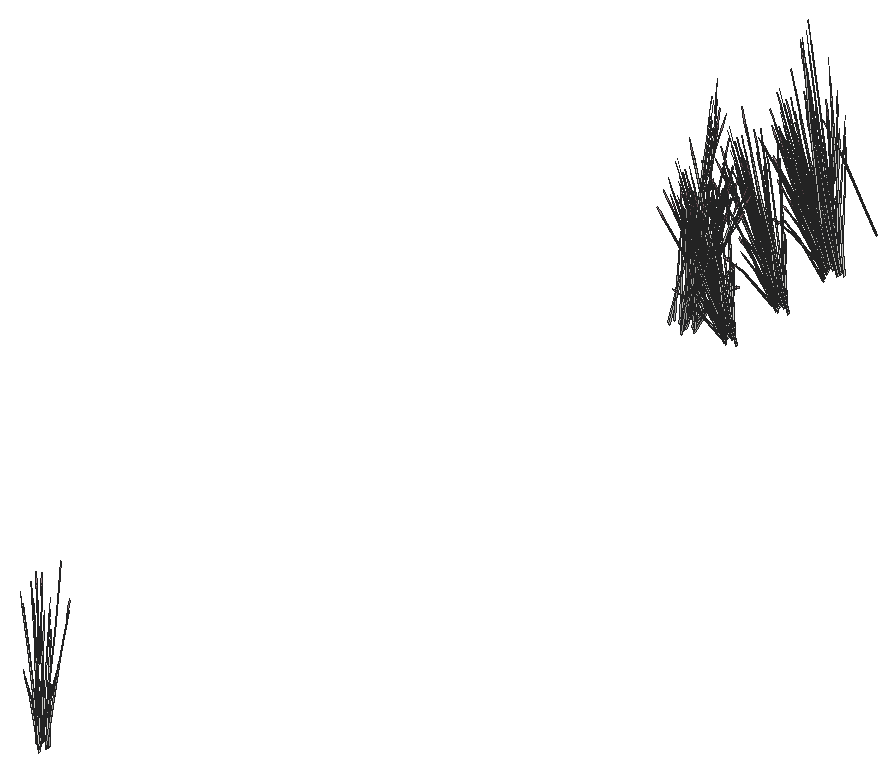
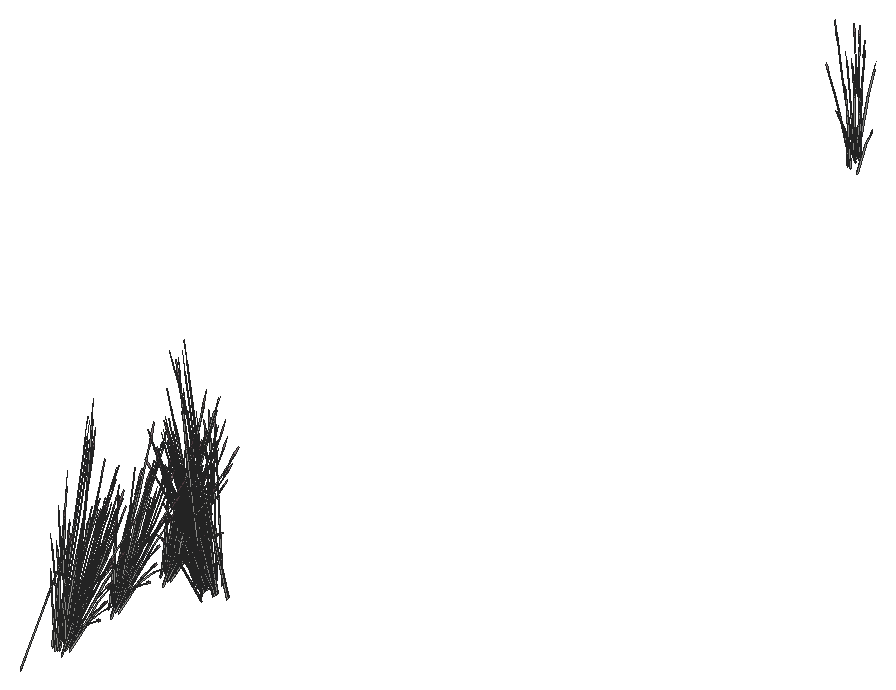
# SketchUp Ruby script. Lengths in inches.
U = 1.inch
M = Sketchup.active_model
def pt(a) = Geom::Point3d.new(a.map { |v| v * U })
def face(e, loops, mat)
  f = e.add_face(loops[0].map { |a| pt(a) })
  loops[1..].each { |l| e.add_face(l.map { |a| pt(a) }).erase! }
  f.material = f.back_material = mat if mat
  f
end
# faces: each face lists its corners as indices into pts; further lists are holes
def faces(e, pts, list, mat = nil) = list.each { |f| face(e, (f[0].is_a?(Array) ? f : [f]).map { |l| l.map { |i| pts[i] } }, mat) }
# xy, xz, yz: faces in a plane at the given z, y or x. An outline is a flat list of corners, or four numbers for a rectangle; further outlines are holes
def ring(l) = l.size == 4 ? [[l[0], l[1]], [l[2], l[1]], [l[2], l[3]], [l[0], l[3]]] : l.each_slice(2).to_a
def flat(e, list, mat, &to3) = list.each { |f| face(e, (f[0].is_a?(Array) ? f : [f]).map { |l| ring(l).map { |u, v| to3.(u, v) } }, mat) }
def xy(e, z, list, mat = nil) = flat(e, list, mat) { |x, y| [x, y, z] }
def xz(e, y, list, mat = nil) = flat(e, list, mat) { |x, z| [x, y, z] }
def yz(e, x, list, mat = nil) = flat(e, list, mat) { |y, z| [x, y, z] }
def lines(e, pts, list) = list.each { |a, b| e.add_line(pt(pts[a]), pt(pts[b])) }
# prism: a flat outline (further loops are holes) pulled along v
def prism(e, loops, v, mat = nil)
  f = face(e, loops, mat); d = Geom::Vector3d.new(v.map { |x| x * U })
  f.pushpull(f.normal.samedirection?(d) ? d.length : -d.length)
end
def box(e, o, s, mat = nil) = prism(e, [[o, [o[0] + s[0], o[1], o[2]], [o[0] + s[0], o[1] + s[1], o[2]], [o[0], o[1] + s[1], o[2]]]], [0, 0, s[2]], mat)
def at(x, y, z, deg = 0) = Geom::Transformation.translation(pt([x, y, z])) * Geom::Transformation.rotation(ORIGIN, Z_AXIS, deg.degrees)
def axes(o, x, y, z) = Geom::Transformation.new([*x, 0, *y, 0, *z, 0, *pt(o).to_a, 1])
def part(name) = M.definitions.add(name)
# library, detail: a bought-in or finely detailed component or shape, given as its bounding box
def library(name, o, s) = part(name).tap { |d| box(d.entities, o, s) }
def detail(e, o, s) = box(e.add_group.entities, o, s)
def put(e, d, t, mat = nil) = e.add_instance(d, t).tap { |i| i.material = mat if mat }
def group(e, t, mat = nil) = e.add_group.tap { |g| g.transformation = t; g.material = mat if mat }.entities
root = M.entities
M.materials.add("LightPink_Translucent").color = [144, 107, 117]
M.materials["LightPink_Translucent"].alpha = 0.75
c1 = part("blade")
p = [[2.15,0.21,22],[0,0.17,0],[0.09,0.45,0],[2.18,0.31,22],[2.29,0.31,22],[0.38,0.45,0],
  [2.48,0.24,33],[2.49,0.24,33],[2.48,0.22,33]]
faces(c1.entities,p,[[0,1,2,3],[4,5,2,3],[6,3,4,7],[8,0,3,6]])
c2 = part("seeds")
p = [[0.3,-0.1,1.38],[-0.01,-0.03,1.59],[-0.01,-0.03,0.03],[0.14,-0.07,-0.07],[0.29,-0.03,3],[0.15,0.01,3.11]]
faces(c2.entities,p,[[0,1,2,3],[1,0,4,5]],"LightPink_Translucent")
c3 = part("blade with seeds")
put(c3.entities,c1,at(0,0,0))
put(c3.entities,c2,axes([2.4,0.25,30.99],[1.5799,-0.05474,1.17369],[-0.12525,1.92788,0.29478],[-0.07173,-0.02425,1.56792]))
put(root,c3,axes([503.15,211.2,4.23],[0.70283,0.33692,-0.1216],[-0.40491,0.48793,-0.67495],[-0.19857,0.16961,1.02557]))
put(root,c3,axes([504.1,211.05,3.07],[0.18977,-0.18775,1.71376],[0.47917,0.50677,0.13857],[-0.32866,0.23079,0.73262]))
put(root,c3,axes([503.5,211.6,3.875],[0.19519,0.55794,-0.51099],[-0.73919,0.0976,-0.3958],[-0.21183,0.14986,0.97773]))
put(root,c3,axes([503.92,212.54,3.92],[-0.62439,-0.02847,0.0643],[0.01712,-0.42991,0.50621],[-0.06534,0.16468,0.77189]))
put(root,c3,axes([502.6,213.03,0.6875],[0.10192,0.06105,1.76342],[0.17281,0.56562,-0.26939],[-0.22588,0.12062,0.30037]))
put(root,c3,axes([504.12,212.57,3.93],[-0.54105,-0.41691,0.48003],[0.57458,-0.35956,0.3958],[-0.0998,0.1956,0.9933]))
put(root,c3,axes([503.96,211.52,3.07],[0.14147,-0.21002,1.71376],[0.59349,0.43464,0.13857],[-0.26773,0.27089,0.73262]))
put(root,c3,axes([504.12,212.7,3.72],[-0.5141,0.32171,-0.35414],[-0.48666,-0.36734,0.4572],[-0.07405,0.18664,0.87481]))
put(root,c3,axes([502.35,212.6,3.91],[-0.01889,0.12092,1.74944],[0.53598,0.42065,-0.27667],[-0.14032,0.19892,0.14031]))
put(root,c3,axes([504.45,213.95,1.96],[-0.01966,-0.36332,1.1486],[0.49135,0.25914,0.84392],[-0.09663,0.17317,0.25299]))
put(root,c3,axes([504.46,212.36,4.53],[-0.01977,0.56521,-0.7886],[-0.83252,-0.03796,0.09517],[-0.08786,0.23945,1.11556]))
put(root,c3,axes([502.29,213.84,3.9],[0.0862,-0.03689,1.77383],[0.71245,0.24539,-0.16761],[-0.01674,0.20431,0.31391]))
put(root,c3,axes([503.875,213.63,1.78],[0.23977,-0.09639,1.43002],[0.59198,0.29065,-0.30754],[-0.1762,0.25149,0.61141]))
put(root,c3,axes([504.19,213.16,2.56],[0.01669,-0.31544,1.54345],[0.75083,0.16661,0.21329],[-0.06506,0.33618,0.72882]))
put(root,c3,axes([493.98,440.93,3.07],[-0.14147,0.21002,1.71376],[-0.59349,-0.43464,0.13857],[0.26773,-0.27089,0.73262]))
put(root,c3,axes([508.48,440.87,4.17],[-0.64788,-0.29534,-0.71045],[0.46044,-0.51755,0.08574],[-0.23473,-0.17635,1.00501]))
put(root,c3,axes([506.8125,441.19,3.07],[0.28223,0.10528,1.71376],[-0.58406,0.44165,0.13857],[-0.36402,-0.19924,0.73262]))
put(root,c3,axes([495.9,440.68,0.6875],[-0.11372,-0.04814,1.76342],[-0.29211,-0.53779,-0.26939],[0.19706,-0.14594,0.30037]))
put(root,c3,axes([508.18,440.88,3.875],[-0.74975,0.14525,-0.51099],[-0.13115,-0.55007,-0.3958],[-0.20138,-0.15763,0.97773]))
put(root,c3,axes([495.25,441,3.93],[0.54105,0.41691,0.48003],[-0.57458,0.35956,0.3958],[0.0998,-0.1956,0.9933]))
put(root,c3,axes([508.7,440.39,4.62],[-0.50709,0.58578,-0.13619],[-0.73436,-0.33748,-0.75594],[-0.25527,-0.1655,1.14864]))
put(root,c3,axes([495.89,442.2,4.17],[0.39688,-0.48213,-0.71045],[0.69548,0.34264,0.08574],[0.23697,-0.17468,1.00501]))
put(root,c3,axes([495.875,441.97,3.875],[-0.19519,-0.55794,-0.51099],[0.73919,-0.0976,-0.3958],[0.21183,-0.14986,0.97773]))
put(root,c3,axes([506.76,440.22,3.91],[-0.16348,-0.00431,1.74944],[-0.52047,0.43131,-0.27667],[-0.2777,-0.08813,0.14031]))
put(root,c3,axes([496.22,442.37,4.23],[-0.70283,-0.33692,-0.1216],[0.40491,-0.48793,-0.67495],[0.19857,-0.16961,1.02557]))
put(root,c3,axes([496.47,441.75,1.78],[-0.27143,-0.0181,1.43002],[-0.27808,-0.48551,-0.30754],[0.33346,-0.13735,0.61141]))
put(root,c3,axes([506.64,441.2,4.29],[0.62747,-0.45094,0.53763],[0.54116,0.47889,0.4433],[-0.29439,-0.08318,1.11249]))
put(root,c3,axes([497.95,442.22,3.9],[-0.09924,-0.00464,1.77383],[-0.4121,-0.49725,-0.16761],[0.1655,-0.1635,0.31391]))
put(root,c3,axes([496.78,440.86,1.96],[-0.25308,0.31105,1.1486],[-0.21753,-0.4179,0.84392],[0.20902,-0.10472,0.25299]))
put(root,c3,axes([496.42,442.03,3.72],[0.66138,-0.08733,-0.35414],[0.17464,0.49921,0.4572],[0.18953,-0.13408,0.87481]))
put(root,c3,axes([506.92,441.2,3.92],[0.03826,-0.46465,0.0643],[0.57772,0.01274,0.50621],[-0.2213,-0.04862,0.77189]))
put(root,c3,axes([506.7,441.34,3.72],[-0.43232,-0.38257,-0.35414],[0.49364,-0.36215,0.4572],[-0.25081,-0.0551,0.87481]))
put(root,c3,axes([495.88,442.32,4.24],[-0.66138,0.08733,0.35414],[-0.17464,-0.49921,-0.4572],[0.18953,-0.13408,0.87481]))
put(root,c3,axes([506.55,441.75,1.78],[0.14835,0.17012,1.43002],[-0.34183,0.46242,-0.30754],[-0.351,-0.11053,0.61141]))
put(root,c3,axes([507.16,441.6,4.17],[-0.75952,-0.01471,-0.71045],[0.05101,-0.61953,0.08574],[-0.32177,-0.06538,1.00501]))
put(root,c3,axes([496.48,442.25,3.92],[0.52161,0.25698,0.0643],[-0.30368,0.36595,0.50621],[0.16723,-0.11831,0.77189]))
put(root,c3,axes([496.33,442.14,3.93],[0.18844,0.56237,0.48003],[-0.73919,0.0976,0.3958],[0.21785,-0.13226,0.9933]))
put(root,c3,axes([498.33,442.82,3.91],[0.10543,-0.09307,1.74944],[-0.13495,-0.57092,-0.27667],[0.26455,-0.10825,0.14031]))
put(root,c3,axes([506.13,440.59,3.9],[0.05633,0.06098,1.77383],[-0.27155,0.54815,-0.16761],[-0.27501,0.00397,0.31391]))
put(root,c3,axes([506.91,441.72,3.875],[-0.55171,0.40476,-0.51099],[-0.48318,-0.42758,-0.3958],[-0.28031,-0.06159,0.97773]))
put(root,c3,axes([507.31,441.54,4.24],[0.43232,0.38257,0.35414],[-0.49364,0.36215,-0.4572],[-0.25081,-0.0551,0.87481]))
put(root,c3,axes([505.66,442.26,1.96],[0.48508,-0.04372,1.1486],[-0.3077,0.38525,0.84392],[-0.23971,-0.05779,0.25299]))
put(root,c3,axes([507.2,441.3,4.23],[-0.04068,0.62141,-0.1216],[-0.77029,-0.01698,-0.67495],[-0.29667,-0.04317,1.02557]))
put(root,c3,axes([496.25,443.69,4.23],[-0.38229,-0.5533,-0.1216],[0.6785,-0.2719,-0.67495],[0.28593,-0.073,1.02557]))
put(root,c3,axes([496.22,443.21,3.875],[0.20584,-0.55581,-0.51099],[0.70573,0.19051,-0.3958],[0.28414,-0.05097,0.97773]))
put(root,c3,axes([495.1,440.95,1.57],[0.47504,-0.61229,0],[0.79476,0.34146,-0.51607],[0.18101,0.07777,1.63711]))
put(root,c3,axes([506.22,442.16,3.07],[0.31515,-0.01384,1.71376],[-0.20907,0.5998,0.13857],[-0.44912,-0.0371,0.73262]))
put(root,c3,axes([496.97,443.37,1.17],[-0.48937,0.07333,1.41583],[-0.07789,-0.58369,0.08104],[0.34275,-0.08835,0.80566]))
put(root,c3,axes([497.86,442.85,1.45],[-0.47106,-0.39072,-0.06488],[0.51591,-0.35801,-0.29416],[0.14618,-0.02521,0.97024]))
put(root,c3,axes([496.08,443.41,4.17],[0.66765,-0.26986,-0.71045],[0.37208,0.55551,0.08574],[0.32259,-0.0631,1.00501]))
put(root,c3,axes([508.56,443.76,1.25],[-0.79037,-0.10018,-0.62353],[0.16679,-0.61794,-0.16365],[-0.23587,-0.07488,1.37633]))
put(root,c3,axes([495.98,443.52,4.24],[-0.63144,-0.17046,0.35414],[0.18417,-0.49731,-0.4572],[0.25423,-0.0456,0.87481]))
put(root,c3,axes([506.09,442.61,3.93],[0.21466,-0.55714,0.48003],[0.70573,0.19051,0.3958],[-0.27753,0.03348,0.9933]))
put(root,c3,axes([491.66,442.03,0.79],[-0.74787,0.24464,1.28929],[-0.23804,-0.70192,0.50096],[0.45924,0.01168,1.46642]))
put(root,c3,axes([506.03,442.46,3.92],[-0.27906,-0.41663,0.0643],[0.50888,-0.20393,0.50621],[-0.22432,0.04024,0.77189]))
put(root,c3,axes([497.5,442.98,0.6875],[-0.03971,-0.09277,1.76342],[0.27541,-0.54264,-0.26939],[0.27782,-0.00781,0.30037]))
put(root,c3,axes([506.02,442.89,0.6875],[0.01927,0.0963,1.76342],[-0.38846,0.5029,-0.26939],[-0.27592,-0.02535,0.30037]))
put(root,c3,axes([493.6,442.39,1.86],[0.76714,-0.40567,-0.29095],[0.51013,0.57321,-0.50002],[0.18927,0.05821,1.59708]))
put(root,c3,axes([496.65,443.46,3.72],[0.63144,0.17046,-0.35414],[-0.18417,0.49731,0.4572],[0.25423,-0.0456,0.87481]))
put(root,c3,axes([495.53,441.32,1.21],[0.7111,0.30552,-0.49651],[-0.42504,0.54784,0],[0.16196,0.06958,1.57504]))
put(root,c3,axes([505.9375,442.67,3.72],[-0.63144,-0.17046,-0.35414],[0.18417,-0.49731,0.4572],[-0.25423,0.0456,0.87481]))
put(root,c3,axes([494.93,442.85,3.07],[-0.31515,0.01384,1.71376],[0.20907,-0.5998,0.13857],[0.44912,0.0371,0.73262]))
put(root,c3,axes([495.34,441.54,1.22],[0.17848,0.53243,-0.30978],[-0.70886,0.15119,0.30978],[0.1429,0.0614,1.38974]))
put(root,c3,axes([496.56,443.67,3.92],[0.27906,0.41663,0.0643],[-0.50888,0.20393,0.50621],[0.22432,-0.04024,0.77189]))
put(root,c3,axes([496.5,443.52,3.93],[-0.21466,0.55714,0.48003],[-0.70573,-0.19051,0.3958],[0.27753,-0.03348,0.9933]))
put(root,c3,axes([506.6,442.62,4.24],[0.63144,0.17046,0.35414],[-0.18417,0.49731,-0.4572],[-0.25423,0.0456,0.87481]))
put(root,c3,axes([507.86,442.59,2.53],[0.21597,-0.08839,1.77064],[0.07448,0.61717,0.13857],[-0.4678,0.08189,0.63284]))
put(root,c3,axes([494.5,442.49,1.25],[0.79037,0.10018,-0.62353],[-0.16679,0.61794,-0.16365],[0.23587,0.07488,1.37633]))
put(root,c3,axes([497.99,443.56,1.96],[-0.46945,0.10088,1.1486],[0.22097,-0.4169,0.84392],[0.24904,0.02853,0.25299]))
put(root,c3,axes([497.77,445.33,3.9],[-0.0687,-0.05349,1.77383],[0.15029,-0.57341,-0.16761],[0.27062,-0.03664,0.31391]))
put(root,c3,axes([505.54,443,3.91],[-0.12407,0.07933,1.74944],[0.01055,0.57963,-0.27667],[-0.2844,0.07538,0.14031]))
put(root,c3,axes([506.37,442.92,3.875],[-0.20584,0.55581,-0.51099],[-0.70573,-0.19051,-0.3958],[-0.28414,0.05097,0.97773]))
put(root,c3,axes([506.34,442.45,4.23],[0.38229,0.5533,-0.1216],[-0.6785,0.2719,-0.67495],[-0.28593,0.073,1.02557]))
put(root,c3,axes([497.17,444.85,3.12],[-0.14542,-0.51365,-0.03492],[0.68734,-0.11809,-0.15832],[0.14353,0.03256,0.52218]))
put(root,c3,axes([495.39,444.83,4.23],[0.04068,-0.62141,-0.1216],[0.77029,0.01698,-0.67495],[0.29667,0.04317,1.02557]))
put(root,c3,axes([495.27,444.59,4.24],[-0.43232,-0.38257,0.35414],[0.49364,-0.36215,-0.4572],[0.25081,0.0551,0.87481]))
put(root,c3,axes([496.0625,444.46,3.91],[0.16299,-0.01033,1.74944],[0.44707,-0.47471,-0.27667],[0.28992,0.06266,0.14031]))
put(root,c3,axes([506.26,444,3.93],[-0.18844,-0.56237,0.48003],[0.73919,-0.0976,0.3958],[-0.21785,0.13226,0.9933]))
put(root,c3,axes([506.11,443.89,3.92],[-0.52161,-0.25698,0.0643],[0.30368,-0.36595,0.50621],[-0.16723,0.11831,0.77189]))
put(root,c3,axes([506.35,443.21,3.07],[0.26363,-0.12925,1.71376],[0.22195,0.59723,0.13857],[-0.41388,0.13498,0.73262]))
put(root,c3,axes([495.43,444.54,4.17],[0.75952,0.01471,-0.71045],[-0.05101,0.61953,0.08574],[0.32177,0.06538,1.00501]))
put(root,c3,axes([505.53,444.23,1.78],[0.26405,0.05016,1.43002],[0.17019,0.51235,-0.30754],[-0.35868,0.0959,0.61141]))
put(root,c3,axes([496.67,443.28,1.57],[0.95008,0,0],[0,0.68292,-0.51607],[0,0.15554,1.63711]))
put(root,c3,axes([504.16,443.59,3.9],[0.09697,0.01639,1.77383],[0.29997,0.53988,-0.16761],[-0.1985,0.1417,0.31391]))
put(root,c3,axes([504.98,445.3,1.96],[0.31665,-0.27694,1.1486],[0.12495,0.43841,0.84392],[-0.22883,0.0785,0.25299]))
put(root,c3,axes([495.89,444.79,3.72],[0.43232,0.38257,-0.35414],[-0.49364,0.36215,0.4572],[0.25081,0.0551,0.87481]))
put(root,c3,axes([495.67,444.9375,3.92],[-0.03826,0.46465,0.0643],[-0.57772,-0.01274,0.50621],[0.2213,0.04862,0.77189]))
put(root,c3,axes([506.17,444.11,3.72],[-0.66138,0.08733,-0.35414],[-0.17464,-0.49921,0.4572],[-0.18953,0.13408,0.87481]))
put(root,c3,axes([495.72,444.79,3.93],[-0.56024,0.40262,0.48003],[-0.48318,-0.42758,0.3958],[0.26285,0.07427,0.9933]))
put(root,c3,axes([494.33,443.81,3.07],[-0.28223,-0.10528,1.71376],[0.58406,-0.44165,0.13857],[0.36402,0.19924,0.73262]))
put(root,c3,axes([493.875,445.51,4.23],[0.45276,-0.52302,-0.1216],[0.65568,0.30132,-0.67495],[0.22792,0.14777,1.02557]))
put(root,c3,axes([507.3125,443.61,3.07],[0.18977,-0.18775,1.71376],[0.47917,0.50677,0.13857],[-0.32866,0.23079,0.73262]))
put(root,c3,axes([506.71,444.16,3.875],[0.19519,0.55794,-0.51099],[-0.73919,0.0976,-0.3958],[-0.21183,0.14986,0.97773]))
put(root,c3,axes([495.5,445.66,0.6875],[0.05536,-0.08822,1.76342],[0.69692,-0.25981,-0.26939],[0.21129,0.13447,0.30037]))
put(root,c3,axes([505.81,445.59,0.6875],[0.10192,0.06105,1.76342],[0.17281,0.56562,-0.26939],[-0.22588,0.12062,0.30037]))
put(root,c3,axes([494.41,445.25,3.875],[0.74975,-0.14525,-0.51099],[0.13115,0.55007,-0.3958],[0.20138,0.15763,0.97773]))
put(root,c3,axes([495.45,445.81,1.86],[-0.48723,-0.01916,1.0506],[0.32177,-0.40701,0.58006],[0.19248,0.1446,0.8241]))
put(root,c3,axes([507.17,444.08,3.07],[0.14147,-0.21002,1.71376],[0.59349,0.43464,0.13857],[-0.26773,0.27089,0.73262]))
put(root,c3,axes([505.5625,445.17,3.91],[-0.01889,0.12092,1.74944],[0.53598,0.42065,-0.27667],[-0.14032,0.19892,0.14031]))
put(root,c3,axes([508.59,458.49,4.17],[-0.64788,-0.29534,-0.71045],[0.46044,-0.51755,0.08574],[-0.23473,-0.17635,1.00501]))
put(root,c3,axes([506.93,458.8125,3.07],[0.28223,0.10528,1.71376],[-0.58406,0.44165,0.13857],[-0.36402,-0.19924,0.73262]))
put(root,c3,axes([508.81,458.01,4.62],[-0.50709,0.58578,-0.13619],[-0.73436,-0.33748,-0.75594],[-0.25527,-0.1655,1.14864]))
put(root,c3,axes([506.87,457.84,3.91],[-0.16348,-0.00431,1.74944],[-0.52047,0.43131,-0.27667],[-0.2777,-0.08813,0.14031]))
put(root,c3,axes([506.75,458.82,4.29],[0.62747,-0.45094,0.53763],[0.54116,0.47889,0.4433],[-0.29439,-0.08318,1.11249]))
put(root,c3,axes([507.04,458.81,3.92],[0.03826,-0.46465,0.0643],[0.57772,0.01274,0.50621],[-0.2213,-0.04862,0.77189]))
put(root,c3,axes([506.82,458.96,3.72],[-0.43232,-0.38257,-0.35414],[0.49364,-0.36215,0.4572],[-0.25081,-0.0551,0.87481]))
put(root,c3,axes([506.66,459.37,1.78],[0.14835,0.17012,1.43002],[-0.34183,0.46242,-0.30754],[-0.351,-0.11053,0.61141]))
put(root,c3,axes([507.27,459.22,4.17],[-0.75952,-0.01471,-0.71045],[0.05101,-0.61953,0.08574],[-0.32177,-0.06538,1.00501]))
put(root,c3,axes([506.24,458.21,3.9],[0.05633,0.06098,1.77383],[-0.27155,0.54815,-0.16761],[-0.27501,0.00397,0.31391]))
put(root,c3,axes([507.02,459.34,3.875],[-0.55171,0.40476,-0.51099],[-0.48318,-0.42758,-0.3958],[-0.28031,-0.06159,0.97773]))
put(root,c3,axes([507.43,459.16,4.24],[0.43232,0.38257,0.35414],[-0.49364,0.36215,-0.4572],[-0.25081,-0.0551,0.87481]))
put(root,c3,axes([505.78,459.88,1.96],[0.48508,-0.04372,1.1486],[-0.3077,0.38525,0.84392],[-0.23971,-0.05779,0.25299]))
put(root,c3,axes([507.3125,458.92,4.23],[-0.04068,0.62141,-0.1216],[-0.77029,-0.01698,-0.67495],[-0.29667,-0.04317,1.02557]))
put(root,c3,axes([506.33,459.77,3.07],[0.31515,-0.01384,1.71376],[-0.20907,0.5998,0.13857],[-0.44912,-0.0371,0.73262]))
put(root,c3,axes([508.67,461.38,1.25],[-0.79037,-0.10018,-0.62353],[0.16679,-0.61794,-0.16365],[-0.23587,-0.07488,1.37633]))
put(root,c3,axes([506.2,460.23,3.93],[0.21466,-0.55714,0.48003],[0.70573,0.19051,0.3958],[-0.27753,0.03348,0.9933]))
put(root,c3,axes([506.15,460.08,3.92],[-0.27906,-0.41663,0.0643],[0.50888,-0.20393,0.50621],[-0.22432,0.04024,0.77189]))
put(root,c3,axes([506.13,460.51,0.6875],[0.01927,0.0963,1.76342],[-0.38846,0.5029,-0.26939],[-0.27592,-0.02535,0.30037]))
put(root,c3,axes([506.05,460.29,3.72],[-0.63144,-0.17046,-0.35414],[0.18417,-0.49731,0.4572],[-0.25423,0.0456,0.87481]))
put(root,c3,axes([506.72,460.23,4.24],[0.63144,0.17046,0.35414],[-0.18417,0.49731,-0.4572],[-0.25423,0.0456,0.87481]))
put(root,c3,axes([507.98,460.21,2.53],[0.21597,-0.08839,1.77064],[0.07448,0.61717,0.13857],[-0.4678,0.08189,0.63284]))
put(root,c3,axes([505.65,460.62,3.91],[-0.12407,0.07933,1.74944],[0.01055,0.57963,-0.27667],[-0.2844,0.07538,0.14031]))
put(root,c3,axes([506.49,460.54,3.875],[-0.20584,0.55581,-0.51099],[-0.70573,-0.19051,-0.3958],[-0.28414,0.05097,0.97773]))
put(root,c3,axes([506.45,460.07,4.23],[0.38229,0.5533,-0.1216],[-0.6785,0.2719,-0.67495],[-0.28593,0.073,1.02557]))
put(root,c3,axes([506.37,461.62,3.93],[-0.18844,-0.56237,0.48003],[0.73919,-0.0976,0.3958],[-0.21785,0.13226,0.9933]))
put(root,c3,axes([506.22,461.51,3.92],[-0.52161,-0.25698,0.0643],[0.30368,-0.36595,0.50621],[-0.16723,0.11831,0.77189]))
put(root,c3,axes([506.46,460.83,3.07],[0.26363,-0.12925,1.71376],[0.22195,0.59723,0.13857],[-0.41388,0.13498,0.73262]))
put(root,c3,axes([505.64,461.85,1.78],[0.26405,0.05016,1.43002],[0.17019,0.51235,-0.30754],[-0.35868,0.0959,0.61141]))
put(root,c3,axes([504.28,461.21,3.9],[0.09697,0.01639,1.77383],[0.29997,0.53988,-0.16761],[-0.1985,0.1417,0.31391]))
put(root,c3,axes([505.09,462.92,1.96],[0.31665,-0.27694,1.1486],[0.12495,0.43841,0.84392],[-0.22883,0.0785,0.25299]))
put(root,c3,axes([506.28,461.72,3.72],[-0.66138,0.08733,-0.35414],[-0.17464,-0.49921,0.4572],[-0.18953,0.13408,0.87481]))
put(root,c3,axes([507.43,461.23,3.07],[0.18977,-0.18775,1.71376],[0.47917,0.50677,0.13857],[-0.32866,0.23079,0.73262]))
put(root,c3,axes([506.83,461.78,3.875],[0.19519,0.55794,-0.51099],[-0.73919,0.0976,-0.3958],[-0.21183,0.14986,0.97773]))
put(root,c3,axes([505.92,463.21,0.6875],[0.10192,0.06105,1.76342],[0.17281,0.56562,-0.26939],[-0.22588,0.12062,0.30037]))
put(root,c3,axes([507.28,461.69,3.07],[0.14147,-0.21002,1.71376],[0.59349,0.43464,0.13857],[-0.26773,0.27089,0.73262]))
put(root,c3,axes([505.67,462.78,3.91],[-0.01889,0.12092,1.74944],[0.53598,0.42065,-0.27667],[-0.14032,0.19892,0.14031]))
put(root,c3,axes([506.04,477.6,3.07],[0.17368,0.19618,1.71376],[-0.80256,0.16516,0.13857],[-0.18139,-0.30799,0.73262]))
put(root,c3,axes([505.82,477.08,1.78],[-0.04601,0.19989,1.43002],[-0.67263,0.16733,-0.30754],[-0.15723,-0.25836,0.61141]))
put(root,c3,axes([506.57,476.02,3.9],[-0.01417,0.07324,1.77383],[-0.6991,0.2658,-0.16761],[-0.20573,-0.13587,0.31391]))
put(root,c3,axes([506.54,477.89,4.17],[-0.64788,-0.29534,-0.71045],[0.46044,-0.51755,0.08574],[-0.23473,-0.17635,1.00501]))
put(root,c3,axes([506.32,477.5,3.72],[-0.11735,-0.49217,-0.35414],[0.67083,-0.12996,0.4572],[-0.18018,-0.14104,0.87481]))
put(root,c3,axes([505.27,477.4,0.6875],[-0.0736,0.08049,1.76342],[-0.74378,0.17355,-0.26939],[-0.17968,-0.15788,0.30037]))
put(root,c3,axes([504.87,478.21,3.07],[0.28223,0.10528,1.71376],[-0.58406,0.44165,0.13857],[-0.36402,-0.19924,0.73262]))
put(root,c3,axes([506.24,477.9,3.875],[-0.74975,0.14525,-0.51099],[-0.13115,-0.55007,-0.3958],[-0.20138,-0.15763,0.97773]))
put(root,c3,axes([506.76,477.41,4.62],[-0.50709,0.58578,-0.13619],[-0.73436,-0.33748,-0.75594],[-0.25527,-0.1655,1.14864]))
put(root,c3,axes([504.82,477.24,3.91],[-0.16348,-0.00431,1.74944],[-0.52047,0.43131,-0.27667],[-0.2777,-0.08813,0.14031]))
put(root,c3,axes([506.71,477.9,4.24],[0.11735,0.49217,0.35414],[-0.67083,0.12996,-0.4572],[-0.18018,-0.14104,0.87481]))
put(root,c3,axes([504.7,478.22,4.29],[0.62747,-0.45094,0.53763],[0.54116,0.47889,0.4433],[-0.29439,-0.08318,1.11249]))
put(root,c3,axes([504.98,478.22,3.92],[0.03826,-0.46465,0.0643],[0.57772,0.01274,0.50621],[-0.2213,-0.04862,0.77189]))
put(root,c3,axes([504.76,478.36,3.72],[-0.43232,-0.38257,-0.35414],[0.49364,-0.36215,0.4572],[-0.25081,-0.0551,0.87481]))
put(root,c3,axes([504.81,477.71,1.32],[-0.21918,0.49894,-0.03893],[-0.6746,-0.15348,-0.17649],[-0.10242,-0.08161,0.58215]))
put(root,c3,axes([504.45,479.99,1.57],[-0.95008,0,0],[0,-0.68292,-0.51607],[0,-0.15554,1.63711]))
put(root,c3,axes([504.61,478.77,1.78],[0.14835,0.17012,1.43002],[-0.34183,0.46242,-0.30754],[-0.351,-0.11053,0.61141]))
put(root,c3,axes([505.22,478.62,4.17],[-0.75952,-0.01471,-0.71045],[0.05101,-0.61953,0.08574],[-0.32177,-0.06538,1.00501]))
put(root,c3,axes([504.1875,477.61,3.9],[0.05633,0.06098,1.77383],[-0.27155,0.54815,-0.16761],[-0.27501,0.00397,0.31391]))
put(root,c3,axes([504.97,478.74,3.875],[-0.55171,0.40476,-0.51099],[-0.48318,-0.42758,-0.3958],[-0.28031,-0.06159,0.97773]))
put(root,c3,axes([505.375,478.5625,4.24],[0.43232,0.38257,0.35414],[-0.49364,0.36215,-0.4572],[-0.25081,-0.0551,0.87481]))
put(root,c3,axes([503.72,479.28,1.96],[0.48508,-0.04372,1.1486],[-0.3077,0.38525,0.84392],[-0.23971,-0.05779,0.25299]))
put(root,c3,axes([505.26,478.32,4.23],[-0.04068,0.62141,-0.1216],[-0.77029,-0.01698,-0.67495],[-0.29667,-0.04317,1.02557]))
put(root,c3,axes([506.62,480.78,1.25],[-0.79037,-0.10018,-0.62353],[0.16679,-0.61794,-0.16365],[-0.23587,-0.07488,1.37633]))
put(root,c3,axes([504.15,479.63,3.93],[0.21466,-0.55714,0.48003],[0.70573,0.19051,0.3958],[-0.27753,0.03348,0.9933]))
put(root,c3,axes([504.09,479.48,3.92],[-0.27906,-0.41663,0.0643],[0.50888,-0.20393,0.50621],[-0.22432,0.04024,0.77189]))
put(root,c3,axes([504.08,479.91,0.6875],[0.01927,0.0963,1.76342],[-0.38846,0.5029,-0.26939],[-0.27592,-0.02535,0.30037]))
put(root,c3,axes([505.78,481.72,1.22],[-0.17848,-0.53243,-0.30978],[0.70886,-0.15119,0.30978],[-0.1429,-0.0614,1.38974]))
put(root,c3,axes([505.58,481.95,1.21],[-0.7111,-0.30552,-0.49651],[0.42504,-0.54784,0],[-0.16196,-0.06958,1.57504]))
put(root,c3,axes([504,479.69,3.72],[-0.63144,-0.17046,-0.35414],[0.18417,-0.49731,0.4572],[-0.25423,0.0456,0.87481]))
put(root,c3,axes([507.52,480.875,1.86],[-0.76714,0.40567,-0.29095],[-0.51013,-0.57321,-0.50002],[-0.18927,-0.05821,1.59708]))
put(root,c3,axes([504.67,479.64,4.24],[0.63144,0.17046,0.35414],[-0.18417,0.49731,-0.4572],[-0.25423,0.0456,0.87481]))
put(root,c3,axes([505.92,479.61,2.53],[0.21597,-0.08839,1.77064],[0.07448,0.61717,0.13857],[-0.4678,0.08189,0.63284]))
put(root,c3,axes([503.6,480.02,3.91],[-0.12407,0.07933,1.74944],[0.01055,0.57963,-0.27667],[-0.2844,0.07538,0.14031]))
put(root,c3,axes([504.43,479.94,3.875],[-0.20584,0.55581,-0.51099],[-0.70573,-0.19051,-0.3958],[-0.28414,0.05097,0.97773]))
put(root,c3,axes([504.4,479.47,4.23],[0.38229,0.5533,-0.1216],[-0.6785,0.2719,-0.67495],[-0.28593,0.073,1.02557]))
put(root,c3,axes([506.02,482.32,1.57],[-0.47504,0.61229,0],[-0.79476,-0.34146,-0.51607],[-0.18101,-0.07777,1.63711]))
put(root,c3,axes([504.32,481.02,3.93],[-0.18844,-0.56237,0.48003],[0.73919,-0.0976,0.3958],[-0.21785,0.13226,0.9933]))
put(root,c3,axes([504.17,480.91,3.92],[-0.52161,-0.25698,0.0643],[0.30368,-0.36595,0.50621],[-0.16723,0.11831,0.77189]))
put(root,c3,axes([504.77,480.83,4.24],[0.66138,-0.08733,0.35414],[0.17464,0.49921,-0.4572],[-0.18953,0.13408,0.87481]))
put(root,c3,axes([502.22,480.61,3.9],[0.09697,0.01639,1.77383],[0.29997,0.53988,-0.16761],[-0.1985,0.1417,0.31391]))
put(root,c3,axes([503.04,482.32,1.96],[0.31665,-0.27694,1.1486],[0.12495,0.43841,0.84392],[-0.22883,0.0785,0.25299]))
put(root,c3,axes([504.23,481.125,3.72],[-0.66138,0.08733,-0.35414],[-0.17464,-0.49921,0.4572],[-0.18953,0.13408,0.87481]))
put(root,c3,axes([503.27,482.25,4.84],[0.67048,0.16311,-0.06488],[-0.20625,0.50201,-0.29416],[-0.10966,0.07622,0.97024]))
put(root,c3,axes([508.03,481.32,1.25],[-0.51177,0.45928,-0.62353],[-0.63575,-0.41646,-0.16365],[-0.20507,0.11457,1.37633]))
put(root,c3,axes([504.43,480.78,4.23],[0.70283,0.33692,-0.1216],[-0.40491,0.48793,-0.67495],[-0.19857,0.16961,1.02557]))
put(root,c3,axes([505.375,480.63,3.07],[0.18977,-0.18775,1.71376],[0.47917,0.50677,0.13857],[-0.32866,0.23079,0.73262]))
put(root,c3,axes([504.78,481.18,3.875],[0.19519,0.55794,-0.51099],[-0.73919,0.0976,-0.3958],[-0.21183,0.14986,0.97773]))
put(root,c3,axes([505.2,482.12,3.92],[-0.62439,-0.02847,0.0643],[0.01712,-0.42991,0.50621],[-0.06534,0.16468,0.77189]))
put(root,c3,axes([503.87,482.61,0.6875],[0.10192,0.06105,1.76342],[0.17281,0.56562,-0.26939],[-0.22588,0.12062,0.30037]))
put(root,c3,axes([505.4,482.16,3.93],[-0.54105,-0.41691,0.48003],[0.57458,-0.35956,0.3958],[-0.0998,0.1956,0.9933]))
put(root,c3,axes([505.23,481.1,3.07],[0.14147,-0.21002,1.71376],[0.59349,0.43464,0.13857],[-0.26773,0.27089,0.73262]))
put(root,c3,axes([505.39,482.28,3.72],[-0.5141,0.32171,-0.35414],[-0.48666,-0.36734,0.4572],[-0.07405,0.18664,0.87481]))
put(root,c3,axes([503.62,482.1875,3.91],[-0.01889,0.12092,1.74944],[0.53598,0.42065,-0.27667],[-0.14032,0.19892,0.14031]))
put(root,c3,axes([505.15,483.21,1.78],[0.23977,-0.09639,1.43002],[0.59198,0.29065,-0.30754],[-0.1762,0.25149,0.61141]))
put(root,c3,axes([504.4,496.52,3.07],[0.17368,0.19618,1.71376],[-0.80256,0.16516,0.13857],[-0.18139,-0.30799,0.73262]))
